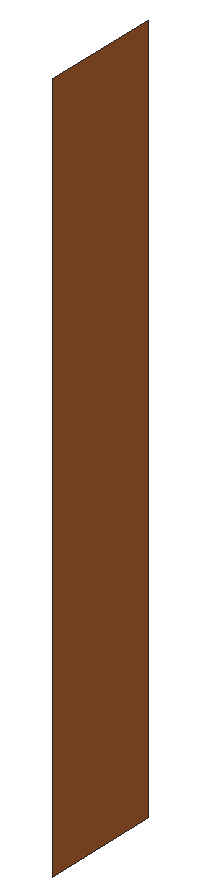
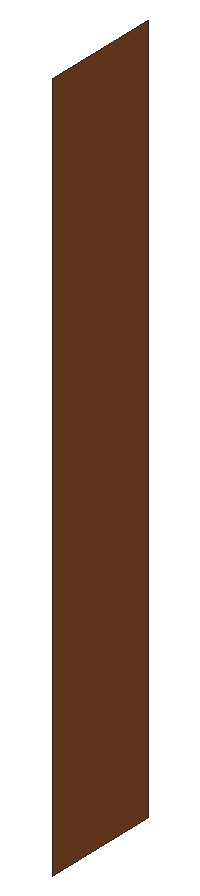
# SketchUp Ruby script. Lengths in inches.
U = 1.inch
M = Sketchup.active_model
def pt(a) = Geom::Point3d.new(a.map { |v| v * U })
def face(e, loops, mat)
  f = e.add_face(loops[0].map { |a| pt(a) })
  loops[1..].each { |l| e.add_face(l.map { |a| pt(a) }).erase! }
  f.material = f.back_material = mat if mat
  f
end
# faces: each face lists its corners as indices into pts; further lists are holes
def faces(e, pts, list, mat = nil) = list.each { |f| face(e, (f[0].is_a?(Array) ? f : [f]).map { |l| l.map { |i| pts[i] } }, mat) }
# xy, xz, yz: faces in a plane at the given z, y or x. An outline is a flat list of corners, or four numbers for a rectangle; further outlines are holes
def ring(l) = l.size == 4 ? [[l[0], l[1]], [l[2], l[1]], [l[2], l[3]], [l[0], l[3]]] : l.each_slice(2).to_a
def flat(e, list, mat, &to3) = list.each { |f| face(e, (f[0].is_a?(Array) ? f : [f]).map { |l| ring(l).map { |u, v| to3.(u, v) } }, mat) }
def xy(e, z, list, mat = nil) = flat(e, list, mat) { |x, y| [x, y, z] }
def xz(e, y, list, mat = nil) = flat(e, list, mat) { |x, z| [x, y, z] }
def yz(e, x, list, mat = nil) = flat(e, list, mat) { |y, z| [x, y, z] }
def lines(e, pts, list) = list.each { |a, b| e.add_line(pt(pts[a]), pt(pts[b])) }
# prism: a flat outline (further loops are holes) pulled along v
def prism(e, loops, v, mat = nil)
  f = face(e, loops, mat); d = Geom::Vector3d.new(v.map { |x| x * U })
  f.pushpull(f.normal.samedirection?(d) ? d.length : -d.length)
end
def box(e, o, s, mat = nil) = prism(e, [[o, [o[0] + s[0], o[1], o[2]], [o[0] + s[0], o[1] + s[1], o[2]], [o[0], o[1] + s[1], o[2]]]], [0, 0, s[2]], mat)
def at(x, y, z, deg = 0) = Geom::Transformation.translation(pt([x, y, z])) * Geom::Transformation.rotation(ORIGIN, Z_AXIS, deg.degrees)
def axes(o, x, y, z) = Geom::Transformation.new([*x, 0, *y, 0, *z, 0, *pt(o).to_a, 1])
def part(name) = M.definitions.add(name)
# library, detail: a bought-in or finely detailed component or shape, given as its bounding box
def library(name, o, s) = part(name).tap { |d| box(d.entities, o, s) }
def detail(e, o, s) = box(e.add_group.entities, o, s)
def put(e, d, t, mat = nil) = e.add_instance(d, t).tap { |i| i.material = mat if mat }
def group(e, t, mat = nil) = e.add_group.tap { |g| g.transformation = t; g.material = mat if mat }.entities
root = M.entities
M.materials.add("[Wood Cherry Original]1").color = [152, 86, 42]
yz(root,445.24,[[178.92,39.83,184.11,71.08]],"[Wood Cherry Original]1")
